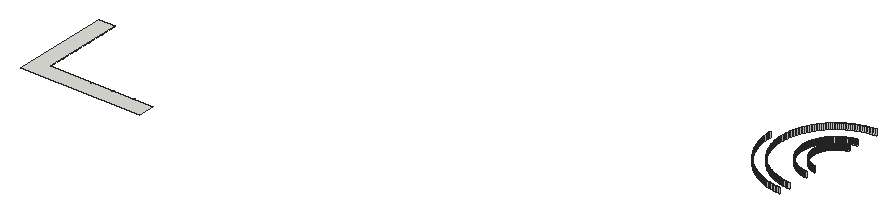
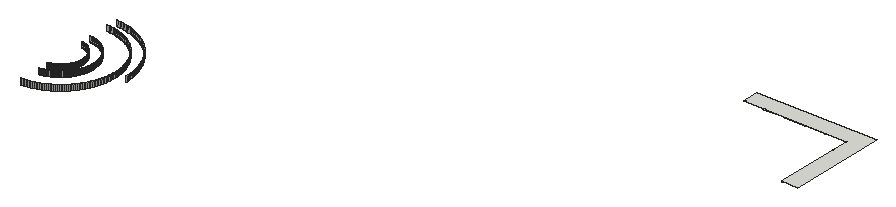
# SketchUp Ruby script. Lengths in inches.
U = 1.inch
M = Sketchup.active_model
def pt(a) = Geom::Point3d.new(a.map { |v| v * U })
def face(e, loops, mat)
  f = e.add_face(loops[0].map { |a| pt(a) })
  loops[1..].each { |l| e.add_face(l.map { |a| pt(a) }).erase! }
  f.material = f.back_material = mat if mat
  f
end
# faces: each face lists its corners as indices into pts; further lists are holes
def faces(e, pts, list, mat = nil) = list.each { |f| face(e, (f[0].is_a?(Array) ? f : [f]).map { |l| l.map { |i| pts[i] } }, mat) }
# xy, xz, yz: faces in a plane at the given z, y or x. An outline is a flat list of corners, or four numbers for a rectangle; further outlines are holes
def ring(l) = l.size == 4 ? [[l[0], l[1]], [l[2], l[1]], [l[2], l[3]], [l[0], l[3]]] : l.each_slice(2).to_a
def flat(e, list, mat, &to3) = list.each { |f| face(e, (f[0].is_a?(Array) ? f : [f]).map { |l| ring(l).map { |u, v| to3.(u, v) } }, mat) }
def xy(e, z, list, mat = nil) = flat(e, list, mat) { |x, y| [x, y, z] }
def xz(e, y, list, mat = nil) = flat(e, list, mat) { |x, z| [x, y, z] }
def yz(e, x, list, mat = nil) = flat(e, list, mat) { |y, z| [x, y, z] }
def lines(e, pts, list) = list.each { |a, b| e.add_line(pt(pts[a]), pt(pts[b])) }
# prism: a flat outline (further loops are holes) pulled along v
def prism(e, loops, v, mat = nil)
  f = face(e, loops, mat); d = Geom::Vector3d.new(v.map { |x| x * U })
  f.pushpull(f.normal.samedirection?(d) ? d.length : -d.length)
end
def box(e, o, s, mat = nil) = prism(e, [[o, [o[0] + s[0], o[1], o[2]], [o[0] + s[0], o[1] + s[1], o[2]], [o[0], o[1] + s[1], o[2]]]], [0, 0, s[2]], mat)
def at(x, y, z, deg = 0) = Geom::Transformation.translation(pt([x, y, z])) * Geom::Transformation.rotation(ORIGIN, Z_AXIS, deg.degrees)
def axes(o, x, y, z) = Geom::Transformation.new([*x, 0, *y, 0, *z, 0, *pt(o).to_a, 1])
def part(name) = M.definitions.add(name)
# library, detail: a bought-in or finely detailed component or shape, given as its bounding box
def library(name, o, s) = part(name).tap { |d| box(d.entities, o, s) }
def detail(e, o, s) = box(e.add_group.entities, o, s)
def put(e, d, t, mat = nil) = e.add_instance(d, t).tap { |i| i.material = mat if mat }
def group(e, t, mat = nil) = e.add_group.tap { |g| g.transformation = t; g.material = mat if mat }.entities
root = M.entities
xy(root,117.11,[[277.82,27,300.22,27.18],[300.625,27,323.02,27.18],[323.42,27,345.82,27.18],[346.22,27,368.625,27.18],[369.02,27,391.42,27.18],
  [277.625,27.2,277.8,44.77],[277.625,45.17,277.8,62.74],[277.625,63.14,277.8,80.71],[277.625,81.11,277.8,98.67],[277.625,99.07,277.8,116.64]])
xy(root,117.3125,[[259.625,9,391.625,9,391.625,27,277.625,27,277.625,116.84,259.625,116.84]])
p = [[902.21,253.35,117.3125],[900.33,253.48,117.3125],[900.33,253.48,111.3125],[902.21,253.35,111.3125],[898.45,253.65,117.3125],[898.45,253.65,111.3125],
  [896.58,253.87,117.3125],[896.58,253.87,111.3125],[894.72,254.14,117.3125],[894.72,254.14,111.3125],[892.86,254.46,117.3125],[892.86,254.46,111.3125],
  [891.01,254.83,117.3125],[891.01,254.83,111.3125],[889.17,255.25,117.3125],[889.17,255.25,111.3125],[887.34,255.71,117.3125],[887.34,255.71,111.3125],
  [885.53,256.22,117.3125],[885.53,256.22,111.3125],[883.73,256.78,117.3125],[883.73,256.78,111.3125],[881.94,257.39,117.3125],[881.94,257.39,111.3125],
  [880.18,258.04,117.3125],[880.18,258.04,111.3125],[878.43,258.74,117.3125],[878.43,258.74,111.3125],[876.69,259.48,117.3125],[876.69,259.48,111.3125],
  [874.98,260.27,117.3125],[874.98,260.27,111.3125],[873.29,261.1,117.3125],[873.29,261.1,111.3125],[871.625,261.98,117.3125],[871.625,261.98,111.3125],
  [869.98,262.9,117.3125],[869.98,262.9,111.3125],[868.36,263.87,117.3125],[868.36,263.87,111.3125],[866.76,264.87,117.3125],[866.76,264.87,111.3125],
  [865.2,265.92,117.3125],[865.2,265.92,111.3125],[901.27,265.44,117.3125],[902.84,265.34,117.3125],[902.84,265.34,111.3125],[901.27,265.44,111.3125],
  [899.71,265.58,117.3125],[899.71,265.58,111.3125],[898.15,265.77,117.3125],[898.15,265.77,111.3125],[896.59,265.99,117.3125],[896.59,265.99,111.3125],
  [863.66,267.01,117.3125],[863.66,267.01,111.3125],[895.04,266.26,117.3125],[895.04,266.26,111.3125],[893.5,266.57,117.3125],[893.5,266.57,111.3125],
  [891.97,266.91,117.3125],[891.97,266.91,111.3125],[890.45,267.3,117.3125],[890.45,267.3,111.3125],[862.15,268.13,117.3125],[862.15,268.13,111.3125],
  [888.9375,267.73,117.3125],[888.9375,267.73,111.3125],[887.4375,268.19,117.3125],[887.4375,268.19,111.3125],[860.67,269.3,117.3125],[860.67,269.3,111.3125],
  [885.95,268.7,117.3125],[885.95,268.7,111.3125],[884.48,269.24,117.3125],[884.48,269.24,111.3125],[883.02,269.82,117.3125],[883.02,269.82,111.3125],
  [859.22,270.51,117.3125],[859.22,270.51,111.3125],[881.57,270.44,117.3125],[881.57,270.44,111.3125],[880.15,271.1,117.3125],[880.15,271.1,111.3125],
  [857.8,271.75,117.3125],[857.8,271.75,111.3125],[878.74,271.8,117.3125],[878.74,271.8,111.3125],[856.42,273.03,117.3125],[856.42,273.03,111.3125],
  [877.35,272.53,117.3125],[877.35,272.53,111.3125],[875.98,273.29,117.3125],[875.98,273.29,111.3125],[855.07,274.34,117.3125],[855.07,274.34,111.3125],
  [874.63,274.1,117.3125],[874.63,274.1,111.3125],[873.3,274.9375,117.3125],[873.3,274.9375,111.3125],[853.75,275.69,117.3125],[853.75,275.69,111.3125],
  [871.99,275.81,117.3125],[871.99,275.81,111.3125],[852.47,277.08,117.3125],[852.47,277.08,111.3125],[870.71,276.72,117.3125],[870.71,276.72,111.3125],
  [869.45,277.66,117.3125],[869.45,277.66,111.3125],[851.23,278.5,117.3125],[851.23,278.5,111.3125],[868.22,278.63,117.3125],[868.22,278.63,111.3125],
  [850.02,279.95,117.3125],[850.02,279.95,111.3125],[867.01,279.63,117.3125],[867.01,279.63,111.3125],[865.83,280.67,117.3125],[865.83,280.67,111.3125],
  [848.86,281.43,117.3125],[848.86,281.43,111.3125],[864.68,281.73,117.3125],[864.68,281.73,111.3125],[847.73,282.9375,117.3125],[847.73,282.9375,111.3125],
  [863.55,282.83,117.3125],[863.55,282.83,111.3125],[862.46,283.95,117.3125],[862.46,283.95,111.3125],[846.64,284.47,117.3125],[846.64,284.47,111.3125],
  [861.39,285.11,117.3125],[861.39,285.11,111.3125],[845.59,286.04,117.3125],[845.59,286.04,111.3125],[860.35,286.29,117.3125],[860.35,286.29,111.3125],
  [844.59,287.64,117.3125],[844.59,287.64,111.3125],[859.35,287.5,117.3125],[859.35,287.5,111.3125],[858.38,288.73,117.3125],[858.38,288.73,111.3125],
  [843.625,289.26,117.3125],[843.625,289.26,111.3125],[857.4375,289.99,117.3125],[857.4375,289.99,111.3125],[842.7,290.9,117.3125],[842.7,290.9,111.3125],
  [902.22,289.45,117.3125],[901.28,289.5625,117.3125],[901.28,289.5625,111.3125],[902.22,289.45,111.3125],[900.35,289.7,117.3125],[900.35,289.7,111.3125],
  [899.42,289.86,117.3125],[899.42,289.86,111.3125],[898.49,290.04,117.3125],[898.49,290.04,111.3125],[856.53,291.27,117.3125],[856.53,291.27,111.3125],
  [897.57,290.25,117.3125],[897.57,290.25,111.3125],[896.66,290.48,117.3125],[896.66,290.48,111.3125],[895.75,290.74,117.3125],[895.75,290.74,111.3125],
  [894.85,291.02,117.3125],[894.85,291.02,111.3125],[841.83,292.57,117.3125],[841.83,292.57,111.3125],[893.96,291.32,117.3125],[893.96,291.32,111.3125],
  [855.66,292.58,117.3125],[855.66,292.58,111.3125],[893.08,291.65,117.3125],[893.08,291.65,111.3125],[892.2,292,117.3125],[892.2,292,111.3125],
  [891.34,292.37,117.3125],[891.34,292.37,111.3125],[890.48,292.76,117.3125],[890.48,292.76,111.3125],[840.99,294.26,117.3125],[840.99,294.26,111.3125],
  [854.82,293.91,117.3125],[854.82,293.91,111.3125],[889.64,293.18,117.3125],[889.64,293.18,111.3125],[888.8,293.62,117.3125],[888.8,293.62,111.3125],
  [887.98,294.08,117.3125],[887.98,294.08,111.3125],[854.02,295.26,117.3125],[854.02,295.26,111.3125],[887.17,294.5625,117.3125],[887.17,294.5625,111.3125],
  [840.2,295.97,117.3125],[840.2,295.97,111.3125],[886.37,295.0625,117.3125],[886.37,295.0625,111.3125],[885.59,295.59,117.3125],[885.59,295.59,111.3125],
  [853.25,296.625,117.3125],[853.25,296.625,111.3125],[884.82,296.13,117.3125],[884.82,296.13,111.3125],[839.46,297.7,117.3125],[839.46,297.7,111.3125],
  [884.0625,296.7,117.3125],[884.0625,296.7,111.3125],[852.52,298.02,117.3125],[852.52,298.02,111.3125],[883.32,297.28,117.3125],[883.32,297.28,111.3125],
  [882.6,297.88,117.3125],[882.6,297.88,111.3125],[838.76,299.45,117.3125],[838.76,299.45,111.3125],[881.89,298.5,117.3125],[881.89,298.5,111.3125],
  [851.82,299.43,117.3125],[851.82,299.43,111.3125],[881.2,299.14,117.3125],[881.2,299.14,111.3125],[880.52,299.8,117.3125],[880.52,299.8,111.3125],
  [851.17,300.85,117.3125],[851.17,300.85,111.3125],[838.11,301.22,117.3125],[838.11,301.22,111.3125],[879.87,300.48,117.3125],[879.87,300.48,111.3125],
  [879.23,301.17,117.3125],[879.23,301.17,111.3125],[850.55,302.3,117.3125],[850.55,302.3,111.3125],[837.5,303.01,117.3125],[837.5,303.01,111.3125],
  [878.6,301.875,117.3125],[878.6,301.875,111.3125],[901.61,301.66,117.3125],[902.22,301.55,117.3125],[902.22,301.55,111.3125],[901.61,301.66,111.3125],
  [900.99,301.78,117.3125],[900.99,301.78,111.3125],[900.375,301.92,117.3125],[900.375,301.92,111.3125],[878,302.6,117.3125],[878,302.6,111.3125],
  [899.77,302.07,117.3125],[899.77,302.07,111.3125],[899.16,302.24,117.3125],[899.16,302.24,111.3125],[898.5625,302.43,117.3125],[898.5625,302.43,111.3125],
  [849.96,303.75,117.3125],[849.96,303.75,111.3125],[897.97,302.63,117.3125],[897.97,302.63,111.3125],[877.42,303.34,117.3125],[877.42,303.34,111.3125],
  [897.38,302.85,117.3125],[897.38,302.85,111.3125],[896.79,303.08,117.3125],[896.79,303.08,111.3125],[836.94,304.81,117.3125],[836.94,304.81,111.3125],
  [896.22,303.33,117.3125],[896.22,303.33,111.3125],[876.85,304.1,117.3125],[876.85,304.1,111.3125],[895.65,303.59,117.3125],[895.65,303.59,111.3125],
  [895.08,303.87,117.3125],[895.08,303.87,111.3125],[849.42,305.23,117.3125],[849.42,305.23,111.3125],[894.53,304.16,117.3125],[894.53,304.16,111.3125],
  [876.31,304.87,117.3125],[876.31,304.87,111.3125],[893.98,304.47,117.3125],[893.98,304.47,111.3125],[893.4375,304.79,117.3125],[893.4375,304.79,111.3125],
  [836.43,306.62,117.3125],[836.43,306.62,111.3125],[892.91,305.13,117.3125],[892.91,305.13,111.3125],[875.79,305.65,117.3125],[875.79,305.65,111.3125],
  [892.38,305.48,117.3125],[892.38,305.48,111.3125],[848.92,306.72,117.3125],[848.92,306.72,111.3125],[891.87,305.84,117.3125],[891.87,305.84,111.3125],
  [875.28,306.45,117.3125],[875.28,306.45,111.3125],[891.37,306.22,117.3125],[891.37,306.22,111.3125],[890.875,306.6,117.3125],[890.875,306.6,111.3125],
  [874.8,307.26,117.3125],[874.8,307.26,111.3125],[835.97,308.45,117.3125],[835.97,308.45,111.3125],[890.39,307.01,117.3125],[890.39,307.01,111.3125],
  [848.45,308.22,117.3125],[848.45,308.22,111.3125],[889.92,307.42,117.3125],[889.92,307.42,111.3125],[874.34,308.08,117.3125],[874.34,308.08,111.3125],
  [889.46,307.85,117.3125],[889.46,307.85,111.3125],[889.01,308.29,117.3125],[889.01,308.29,111.3125],[873.9,308.91,117.3125],[873.9,308.91,111.3125],
  [848.02,309.73,117.3125],[848.02,309.73,111.3125],[888.57,308.74,117.3125],[888.57,308.74,111.3125],[835.55,310.29,117.3125],[835.55,310.29,111.3125],
  [888.14,309.2,117.3125],[888.14,309.2,111.3125],[873.49,309.76,117.3125],[873.49,309.76,111.3125],[887.73,309.67,117.3125],[887.73,309.67,111.3125],
  [847.64,311.25,117.3125],[847.64,311.25,111.3125],[887.33,310.15,117.3125],[887.33,310.15,111.3125],[873.09,310.61,117.3125],[873.09,310.61,111.3125],
  [886.9375,310.65,117.3125],[886.9375,310.65,111.3125],[835.18,312.14,117.3125],[835.18,312.14,111.3125],[872.72,311.48,117.3125],[872.72,311.48,111.3125],
  [886.5625,311.15,117.3125],[886.5625,311.15,111.3125],[886.2,311.66,117.3125],[886.2,311.66,111.3125],[847.29,312.78,117.3125],[847.29,312.78,111.3125],
  [872.37,312.35,117.3125],[872.37,312.35,111.3125],[885.85,312.18,117.3125],[885.85,312.18,111.3125],[834.87,313.99,117.3125],[834.87,313.99,111.3125],
  [885.52,312.72,117.3125],[885.52,312.72,111.3125],[872.04,313.24,117.3125],[872.04,313.24,111.3125],[885.19,313.26,117.3125],[885.19,313.26,111.3125],
  [846.98,314.32,117.3125],[846.98,314.32,111.3125],[871.74,314.13,117.3125],[871.74,314.13,111.3125],[884.89,313.8,117.3125],[884.89,313.8,111.3125],
  [884.59,314.36,117.3125],[884.59,314.36,111.3125],[834.59,315.86,117.3125],[834.59,315.86,111.3125],[871.46,315.03,117.3125],[871.46,315.03,111.3125],
  [846.72,315.87,117.3125],[846.72,315.87,111.3125],[884.32,314.92,117.3125],[884.32,314.92,111.3125],[884.05,315.49,117.3125],[884.05,315.49,111.3125],
  [871.21,315.9375,117.3125],[871.21,315.9375,111.3125],[883.81,316.07,117.3125],[883.81,316.07,111.3125],[834.375,317.73,117.3125],[834.375,317.73,111.3125],
  [846.49,317.42,117.3125],[846.49,317.42,111.3125],[870.97,316.85,117.3125],[870.97,316.85,111.3125],[883.57,316.66,117.3125],[883.57,316.66,111.3125],
  [883.36,317.24,117.3125],[883.36,317.24,111.3125],[870.77,317.77,117.3125],[870.77,317.77,111.3125],[883.15,317.84,117.3125],[883.15,317.84,111.3125],
  [846.31,318.98,117.3125],[846.31,318.98,111.3125],[834.2,319.61,117.3125],[834.2,319.61,111.3125],[870.58,318.7,117.3125],[870.58,318.7,111.3125],
  [882.97,318.44,117.3125],[882.97,318.44,111.3125],[882.8,319.04,117.3125],[882.8,319.04,111.3125],[870.42,319.625,117.3125],[870.42,319.625,111.3125],
  [846.16,320.55,117.3125],[846.16,320.55,111.3125],[882.64,319.65,117.3125],[882.64,319.65,111.3125],[834.08,321.49,117.3125],[834.08,321.49,111.3125],
  [870.29,320.56,117.3125],[870.29,320.56,111.3125],[882.5,320.27,117.3125],[882.5,320.27,111.3125],[882.38,320.88,117.3125],[882.38,320.88,111.3125],
  [846.0625,322.12,117.3125],[846.0625,322.12,111.3125],[870.18,321.49,117.3125],[870.18,321.49,111.3125],[882.27,321.5,117.3125],[882.27,321.5,111.3125],
  [834,323.37,117.3125],[834,323.37,111.3125],[870.09,322.43,117.3125],[870.09,322.43,111.3125],[882.18,322.125,117.3125],[882.18,322.125,111.3125],
  [846,323.6875,117.3125],[846,323.6875,111.3125],[882.11,322.75,117.3125],[882.11,322.75,111.3125],[870.03,323.37,117.3125],[870.03,323.37,111.3125],
  [882.05,323.375,117.3125],[882.05,323.375,111.3125],[833.98,325.26,117.3125],[833.98,325.26,111.3125],[869.99,324.3125,117.3125],[869.99,324.3125,111.3125],
  [882.01,324,117.3125],[882.01,324,111.3125],[845.98,325.26,117.3125],[845.98,325.26,111.3125],[881.99,324.63,117.3125],[881.99,324.63,111.3125],
  [869.98,325.26,117.3125],[869.98,325.26,111.3125],[881.98,325.26,117.3125],[881.98,325.26,111.3125],[846,326.83,117.3125],[846,326.83,111.3125],
  [869.99,326.2,117.3125],[869.99,326.2,111.3125],[881.99,325.88,117.3125],[881.99,325.88,111.3125],[882.01,326.51,117.3125],[882.01,326.51,111.3125],
  [870.03,327.14,117.3125],[870.03,327.14,111.3125],[882.05,327.14,117.3125],[882.05,327.14,111.3125],[846.0625,328.4,117.3125],[846.0625,328.4,111.3125],
  [870.09,328.08,117.3125],[870.09,328.08,111.3125],[882.11,327.76,117.3125],[882.11,327.76,111.3125],[882.18,328.39,117.3125],[882.18,328.39,111.3125],
  [870.18,329.02,117.3125],[870.18,329.02,111.3125],[846.16,329.96,117.3125],[846.16,329.96,111.3125],[882.27,329.01,117.3125],[882.27,329.01,111.3125],
  [870.29,329.96,117.3125],[870.29,329.96,111.3125],[882.38,329.63,117.3125],[882.38,329.63,111.3125],[882.5,330.25,117.3125],[882.5,330.25,111.3125],
  [846.31,331.53,117.3125],[846.31,331.53,111.3125],[870.42,330.89,117.3125],[870.42,330.89,111.3125],[882.64,330.86,117.3125],[882.64,330.86,111.3125],
  [870.58,331.82,117.3125],[870.58,331.82,111.3125],[882.8,331.47,117.3125],[882.8,331.47,111.3125],[846.49,333.09,117.3125],[846.49,333.09,111.3125],
  [882.97,332.07,117.3125],[882.97,332.07,111.3125],[870.77,332.74,117.3125],[870.77,332.74,111.3125],[883.15,332.67,117.3125],[883.15,332.67,111.3125],
  [870.97,333.66,117.3125],[870.97,333.66,111.3125],[883.36,333.27,117.3125],[883.36,333.27,111.3125],[846.72,334.64,117.3125],[846.72,334.64,111.3125],
  [883.57,333.86,117.3125],[883.57,333.86,111.3125],[871.21,334.57,117.3125],[871.21,334.57,111.3125],[883.81,334.44,117.3125],[883.81,334.44,111.3125],
  [884.05,335.02,117.3125],[884.05,335.02,111.3125],[846.98,336.19,117.3125],[846.98,336.19,111.3125],[871.46,335.48,117.3125],[871.46,335.48,111.3125],
  [884.32,335.59,117.3125],[884.32,335.59,111.3125],[871.74,336.38,117.3125],[871.74,336.38,111.3125],[884.59,336.15,117.3125],[884.59,336.15,111.3125],
  [847.29,337.73,117.3125],[847.29,337.73,111.3125],[884.89,336.71,117.3125],[884.89,336.71,111.3125],[872.04,337.27,117.3125],[872.04,337.27,111.3125],
  [885.19,337.26,117.3125],[885.19,337.26,111.3125],[872.37,338.16,117.3125],[872.37,338.16,111.3125],[885.52,337.8,117.3125],[885.52,337.8,111.3125],
  [847.64,339.26,117.3125],[847.64,339.26,111.3125],[885.85,338.33,117.3125],[885.85,338.33,111.3125],[872.72,339.03,117.3125],[872.72,339.03,111.3125],
  [886.2,338.85,117.3125],[886.2,338.85,111.3125],[886.5625,339.36,117.3125],[886.5625,339.36,111.3125],[873.09,339.9,117.3125],[873.09,339.9,111.3125],
  [848.02,340.79,117.3125],[848.02,340.79,111.3125],[886.9375,339.87,117.3125],[886.9375,339.87,111.3125],[873.49,340.75,117.3125],[873.49,340.75,111.3125],
  [887.33,340.36,117.3125],[887.33,340.36,111.3125],[887.73,340.84,117.3125],[887.73,340.84,111.3125],[848.45,342.3,117.3125],[848.45,342.3,111.3125],
  [873.9,341.6,117.3125],[873.9,341.6,111.3125],[888.14,341.32,117.3125],[888.14,341.32,111.3125],[888.57,341.78,117.3125],[888.57,341.78,111.3125],
  [874.34,342.43,117.3125],[874.34,342.43,111.3125],[889.01,342.23,117.3125],[889.01,342.23,111.3125],[889.46,342.67,117.3125],[889.46,342.67,111.3125],
  [848.92,343.8,117.3125],[848.92,343.8,111.3125],[874.8,343.26,117.3125],[874.8,343.26,111.3125],[889.92,343.09,117.3125],[889.92,343.09,111.3125],
  [890.39,343.51,117.3125],[890.39,343.51,111.3125],[875.28,344.07,117.3125],[875.28,344.07,111.3125],[890.875,343.91,117.3125],[890.875,343.91,111.3125],
  [849.42,345.28,117.3125],[849.42,345.28,111.3125],[891.37,344.3,117.3125],[891.37,344.3,111.3125],[875.79,344.86,117.3125],[875.79,344.86,111.3125],
  [891.87,344.67,117.3125],[891.87,344.67,111.3125],[892.38,345.04,117.3125],[892.38,345.04,111.3125],[876.31,345.65,117.3125],[876.31,345.65,111.3125],
  [892.91,345.38,117.3125],[892.91,345.38,111.3125],[849.96,346.76,117.3125],[849.96,346.76,111.3125],[893.4375,345.72,117.3125],[893.4375,345.72,111.3125],
  [876.85,346.42,117.3125],[876.85,346.42,111.3125],[893.98,346.04,117.3125],[893.98,346.04,111.3125],[894.53,346.35,117.3125],[894.53,346.35,111.3125],
  [895.08,346.64,117.3125],[895.08,346.64,111.3125],[877.42,347.17,117.3125],[877.42,347.17,111.3125],[895.65,346.92,117.3125],[895.65,346.92,111.3125],
  [850.55,348.22,117.3125],[850.55,348.22,111.3125],[896.22,347.18,117.3125],[896.22,347.18,111.3125],[878,347.91,117.3125],[878,347.91,111.3125],
  [896.79,347.43,117.3125],[896.79,347.43,111.3125],[897.38,347.66,117.3125],[897.38,347.66,111.3125],[897.97,347.88,117.3125],[897.97,347.88,111.3125],
  [878.6,348.64,117.3125],[878.6,348.64,111.3125],[898.5625,348.08,117.3125],[898.5625,348.08,111.3125],[899.16,348.27,117.3125],[899.16,348.27,111.3125],
  [851.17,349.66,117.3125],[851.17,349.66,111.3125],[899.77,348.4375,117.3125],[899.77,348.4375,111.3125],[900.375,348.59,117.3125],[900.375,348.59,111.3125],
  [879.23,349.34,117.3125],[879.23,349.34,111.3125],[900.99,348.73,117.3125],[900.99,348.73,111.3125],[901.61,348.85,117.3125],[901.61,348.85,111.3125],
  [902.22,348.96,117.3125],[902.22,348.96,111.3125],[879.87,350.04,117.3125],[879.87,350.04,111.3125],[851.82,351.09,117.3125],[851.82,351.09,111.3125],
  [880.52,350.71,117.3125],[880.52,350.71,111.3125],[881.2,351.37,117.3125],[881.2,351.37,111.3125],[852.52,352.5,117.3125],[852.52,352.5,111.3125],
  [881.89,352.01,117.3125],[881.89,352.01,111.3125],[882.6,352.63,117.3125],[882.6,352.63,111.3125],[853.25,353.89,117.3125],[853.25,353.89,111.3125],
  [883.32,353.23,117.3125],[883.32,353.23,111.3125],[884.0625,353.82,117.3125],[884.0625,353.82,111.3125],[884.82,354.38,117.3125],[884.82,354.38,111.3125],
  [854.02,355.26,117.3125],[854.02,355.26,111.3125],[885.59,354.92,117.3125],[885.59,354.92,111.3125],[886.37,355.45,117.3125],[886.37,355.45,111.3125],
  [854.82,356.61,117.3125],[854.82,356.61,111.3125],[887.17,355.95,117.3125],[887.17,355.95,111.3125],[887.98,356.43,117.3125],[887.98,356.43,111.3125],
  [888.8,356.89,117.3125],[888.8,356.89,111.3125],[855.66,357.93,117.3125],[855.66,357.93,111.3125],[889.64,357.33,117.3125],[889.64,357.33,111.3125],
  [890.48,357.75,117.3125],[890.48,357.75,111.3125],[891.34,358.14,117.3125],[891.34,358.14,111.3125],[856.53,359.24,117.3125],[856.53,359.24,111.3125],
  [892.2,358.52,117.3125],[892.2,358.52,111.3125],[893.08,358.87,117.3125],[893.08,358.87,111.3125],[893.96,359.19,117.3125],[893.96,359.19,111.3125],
  [857.4375,360.52,117.3125],[857.4375,360.52,111.3125],[894.85,359.49,117.3125],[894.85,359.49,111.3125],[895.75,359.77,117.3125],[895.75,359.77,111.3125],
  [896.66,360.03,117.3125],[896.66,360.03,111.3125],[897.57,360.26,117.3125],[897.57,360.26,111.3125],[898.49,360.47,117.3125],[898.49,360.47,111.3125],
  [858.38,361.78,117.3125],[858.38,361.78,111.3125],[899.42,360.65,117.3125],[899.42,360.65,111.3125],[900.35,360.8125,117.3125],[900.35,360.8125,111.3125],
  [901.28,360.95,117.3125],[901.28,360.95,111.3125],[902.22,361.06,117.3125],[902.22,361.06,111.3125],[859.35,363.02,117.3125],[859.35,363.02,111.3125],
  [860.35,364.22,117.3125],[860.35,364.22,111.3125],[861.39,365.4,117.3125],[861.39,365.4,111.3125],[862.46,366.56,117.3125],[862.46,366.56,111.3125],
  [863.55,367.68,117.3125],[863.55,367.68,111.3125],[864.68,368.78,117.3125],[864.68,368.78,111.3125],[865.83,369.84,117.3125],[865.83,369.84,111.3125],
  [867.01,370.88,117.3125],[867.01,370.88,111.3125],[868.22,371.88,117.3125],[868.22,371.88,111.3125],[869.45,372.86,117.3125],[869.45,372.86,111.3125],
  [870.71,373.8,117.3125],[870.71,373.8,111.3125],[871.99,374.7,117.3125],[871.99,374.7,111.3125],[873.3,375.58,117.3125],[873.3,375.58,111.3125],
  [874.63,376.41,117.3125],[874.63,376.41,111.3125],[875.98,377.22,117.3125],[875.98,377.22,111.3125],[877.35,377.99,117.3125],[877.35,377.99,111.3125],
  [878.74,378.72,117.3125],[878.74,378.72,111.3125],[880.15,379.41,117.3125],[880.15,379.41,111.3125],[881.57,380.07,117.3125],[881.57,380.07,111.3125],
  [883.02,380.6875,117.3125],[883.02,380.6875,111.3125],[884.48,381.27,117.3125],[884.48,381.27,111.3125],[885.95,381.81,117.3125],[885.95,381.81,111.3125],
  [887.4375,382.32,117.3125],[887.4375,382.32,111.3125],[888.9375,382.79,117.3125],[888.9375,382.79,111.3125],[890.45,383.21,117.3125],[890.45,383.21,111.3125],
  [891.97,383.6,117.3125],[891.97,383.6,111.3125],[893.5,383.95,117.3125],[893.5,383.95,111.3125],[895.04,384.25,117.3125],[895.04,384.25,111.3125],
  [896.59,384.52,117.3125],[896.59,384.52,111.3125],[898.15,384.74,117.3125],[898.15,384.74,111.3125],[899.71,384.93,117.3125],[899.71,384.93,111.3125],
  [901.27,385.07,117.3125],[901.27,385.07,111.3125],[902.84,385.17,117.3125],[902.84,385.17,111.3125]]
faces(root,p,[[0,1,2,3],[1,4,5,2],[4,6,7,5],[6,8,9,7],[8,10,11,9],[10,12,13,11],[12,14,15,13],[14,16,17,15],
  [16,18,19,17],[18,20,21,19],[20,22,23,21],[22,24,25,23],[24,26,27,25],[26,28,29,27],[28,30,31,29],[30,32,33,31],
  [32,34,35,33],[34,36,37,35],[36,38,39,37],[38,40,41,39],[40,42,43,41],[44,45,46,47],[48,44,47,49],[50,48,49,51],
  [52,50,51,53],[42,54,55,43],[56,52,53,57],[58,56,57,59],[60,58,59,61],[62,60,61,63],[54,64,65,55],[66,62,63,67],
  [68,66,67,69],[64,70,71,65],[72,68,69,73],[74,72,73,75],[76,74,75,77],[70,78,79,71],[80,76,77,81],[82,80,81,83],
  [78,84,85,79],[86,82,83,87],[84,88,89,85],[90,86,87,91],[92,90,91,93],[88,94,95,89],[96,92,93,97],[98,96,97,99],
  [94,100,101,95],[102,98,99,103],[100,104,105,101],[106,102,103,107],[108,106,107,109],[104,110,111,105],[112,108,109,113],[110,114,115,111],
  [116,112,113,117],[118,116,117,119],[114,120,121,115],[122,118,119,123],[120,124,125,121],[126,122,123,127],[128,126,127,129],[124,130,131,125],
  [132,128,129,133],[130,134,135,131],[136,132,133,137],[134,138,139,135],[140,136,137,141],[142,140,141,143],[138,144,145,139],[146,142,143,147],
  [144,148,149,145],[150,151,152,153],[151,154,155,152],[154,156,157,155],[156,158,159,157],[160,146,147,161],[158,162,163,159],[162,164,165,163],
  [164,166,167,165],[166,168,169,167],[148,170,171,149],[168,172,173,169],[174,160,161,175],[172,176,177,173],[176,178,179,177],[178,180,181,179],
  [180,182,183,181],[170,184,185,171],[186,174,175,187],[182,188,189,183],[188,190,191,189],[190,192,193,191],[194,186,187,195],[192,196,197,193],
  [184,198,199,185],[196,200,201,197],[200,202,203,201],[204,194,195,205],[202,206,207,203],[198,208,209,199],[206,210,211,207],[212,204,205,213],
  [210,214,215,211],[214,216,217,215],[208,218,219,209],[216,220,221,217],[222,212,213,223],[220,224,225,221],[224,226,227,225],[228,222,223,229],
  [218,230,231,219],[226,232,233,227],[232,234,235,233],[236,228,229,237],[230,238,239,231],[234,240,241,235],[242,243,244,245],[246,242,245,247],
  [248,246,247,249],[240,250,251,241],[252,248,249,253],[254,252,253,255],[256,254,255,257],[258,236,237,259],[260,256,257,261],[250,262,263,251],
  [264,260,261,265],[266,264,265,267],[238,268,269,239],[270,266,267,271],[262,272,273,263],[274,270,271,275],[276,274,275,277],[278,258,259,279],
  [280,276,277,281],[272,282,283,273],[284,280,281,285],[286,284,285,287],[268,288,289,269],[290,286,287,291],[282,292,293,283],[294,290,291,295],
  [296,278,279,297],[298,294,295,299],[292,300,301,293],[302,298,299,303],[304,302,303,305],[300,306,307,301],[288,308,309,289],[310,304,305,311],
  [312,296,297,313],[314,310,311,315],[306,316,317,307],[318,314,315,319],[320,318,319,321],[316,322,323,317],[324,312,313,325],[326,320,321,327],
  [308,328,329,309],[330,326,327,331],[322,332,333,323],[334,330,331,335],[336,324,325,337],[338,334,335,339],[332,340,341,333],[342,338,339,343],
  [328,344,345,329],[340,346,347,341],[348,342,343,349],[350,348,349,351],[352,336,337,353],[346,354,355,347],[356,350,351,357],[344,358,359,345],
  [360,356,357,361],[354,362,363,355],[364,360,361,365],[366,352,353,367],[362,368,369,363],[370,364,365,371],[372,370,371,373],[358,374,375,359],
  [368,376,377,369],[378,366,367,379],[380,372,373,381],[382,380,381,383],[376,384,385,377],[386,382,383,387],[374,388,389,375],[390,378,379,391],
  [384,392,393,385],[394,386,387,395],[396,394,395,397],[392,398,399,393],[400,396,397,401],[402,390,391,403],[388,404,405,389],[398,406,407,399],
  [408,400,401,409],[410,408,409,411],[406,412,413,407],[414,402,403,415],[416,410,411,417],[404,418,419,405],[412,420,421,413],[422,416,417,423],
  [424,422,423,425],[426,414,415,427],[420,428,429,421],[430,424,425,431],[418,432,433,419],[428,434,435,429],[436,430,431,437],[438,426,427,439],
  [440,436,437,441],[434,442,443,435],[444,440,441,445],[432,446,447,433],[442,448,449,443],[450,444,445,451],[452,438,439,453],[454,450,451,455],
  [448,456,457,449],[458,454,455,459],[460,452,453,461],[456,462,463,457],[464,458,459,465],[466,464,465,467],[462,468,469,463],[470,466,467,471],
  [472,460,461,473],[468,474,475,469],[476,470,471,477],[478,476,477,479],[474,480,481,475],[482,472,473,483],[484,478,479,485],[480,486,487,481],
  [488,484,485,489],[490,488,489,491],[492,482,483,493],[486,494,495,487],[496,490,491,497],[494,498,499,495],[500,496,497,501],[502,492,493,503],
  [504,500,501,505],[498,506,507,499],[508,504,505,509],[506,510,511,507],[512,508,509,513],[514,502,503,515],[516,512,513,517],[510,518,519,511],
  [520,516,517,521],[522,520,521,523],[524,514,515,525],[518,526,527,519],[528,522,523,529],[526,530,531,527],[532,528,529,533],[534,524,525,535],
  [536,532,533,537],[530,538,539,531],[540,536,537,541],[538,542,543,539],[544,540,541,545],[546,534,535,547],[548,544,545,549],[542,550,551,543],
  [552,548,549,553],[554,552,553,555],[550,556,557,551],[558,546,547,559],[560,554,555,561],[556,562,563,557],[564,560,561,565],[566,564,565,567],
  [568,558,559,569],[562,570,571,563],[572,566,567,573],[574,572,573,575],[570,576,577,571],[578,574,575,579],[580,578,579,581],[582,568,569,583],
  [576,584,585,577],[586,580,581,587],[588,586,587,589],[584,590,591,585],[592,588,589,593],[594,582,583,595],[596,592,593,597],[590,598,599,591],
  [600,596,597,601],[602,600,601,603],[598,604,605,599],[606,602,603,607],[608,594,595,609],[610,606,607,611],[604,612,613,605],[614,610,611,615],
  [616,614,615,617],[618,616,617,619],[612,620,621,613],[622,618,619,623],[624,608,609,625],[626,622,623,627],[620,628,629,621],[630,626,627,631],
  [632,630,631,633],[634,632,633,635],[628,636,637,629],[638,634,635,639],[640,638,639,641],[642,624,625,643],[644,640,641,645],[646,644,645,647],
  [636,648,649,637],[650,646,647,651],[652,650,651,653],[654,652,653,655],[648,656,657,649],[658,642,643,659],[656,660,661,657],[660,662,663,661],
  [664,658,659,665],[662,666,667,663],[666,668,669,667],[670,664,665,671],[668,672,673,669],[672,674,675,673],[674,676,677,675],[678,670,671,679],
  [676,680,681,677],[680,682,683,681],[684,678,679,685],[682,686,687,683],[686,688,689,687],[688,690,691,689],[692,684,685,693],[690,694,695,691],
  [694,696,697,695],[696,698,699,697],[700,692,693,701],[698,702,703,699],[702,704,705,703],[704,706,707,705],[708,700,701,709],[706,710,711,707],
  [710,712,713,711],[712,714,715,713],[714,716,717,715],[716,718,719,717],[720,708,709,721],[718,722,723,719],[722,724,725,723],[724,726,727,725],
  [726,728,729,727],[730,720,721,731],[732,730,731,733],[734,732,733,735],[736,734,735,737],[738,736,737,739],[740,738,739,741],[742,740,741,743],
  [744,742,743,745],[746,744,745,747],[748,746,747,749],[750,748,749,751],[752,750,751,753],[754,752,753,755],[756,754,755,757],[758,756,757,759],
  [760,758,759,761],[762,760,761,763],[764,762,763,765],[766,764,765,767],[768,766,767,769],[770,768,769,771],[772,770,771,773],[774,772,773,775],
  [776,774,775,777],[778,776,777,779],[780,778,779,781],[782,780,781,783],[784,782,783,785],[786,784,785,787],[788,786,787,789],[790,788,789,791],
  [792,790,791,793],[794,792,793,795]])
